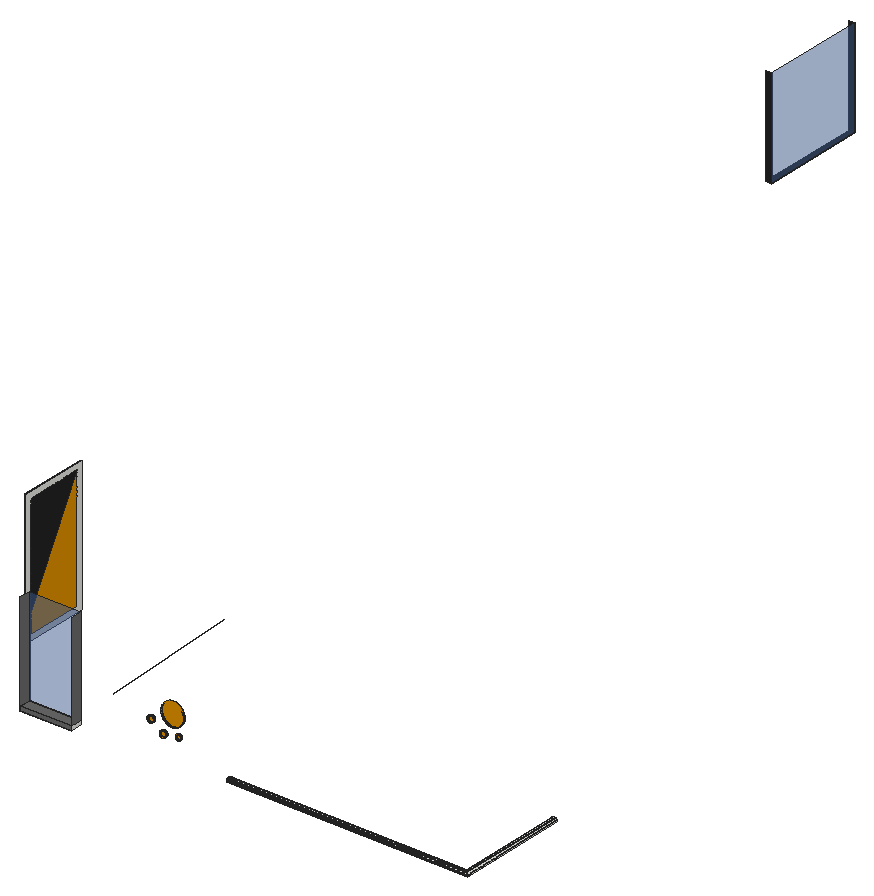
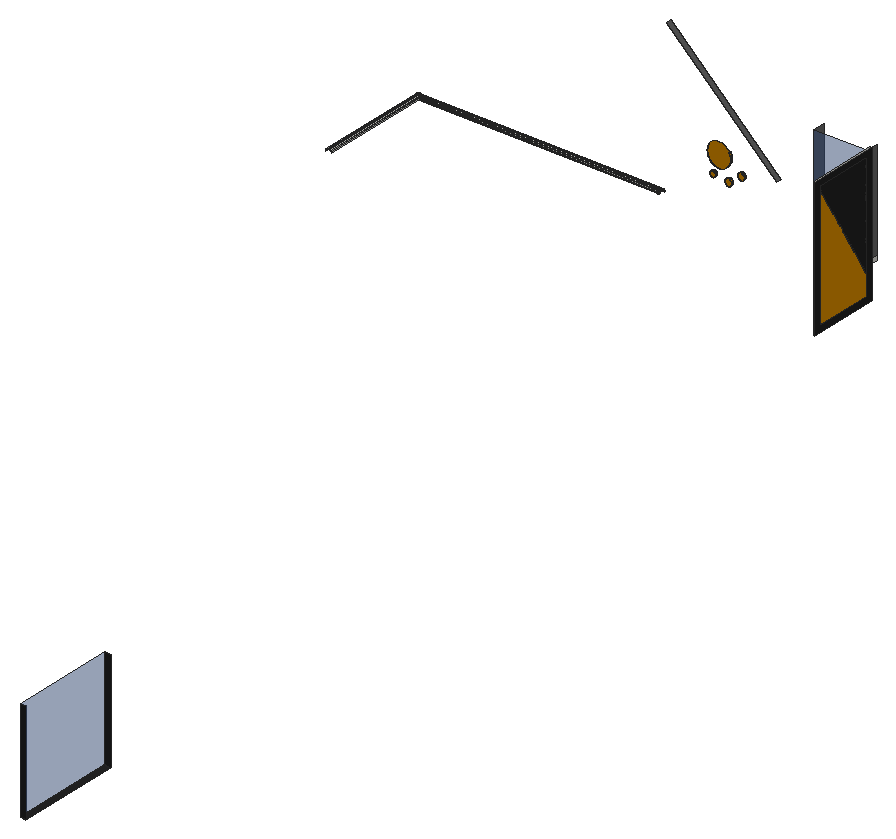
# SketchUp Ruby script. Lengths in inches.
U = 1.inch
M = Sketchup.active_model
def pt(a) = Geom::Point3d.new(a.map { |v| v * U })
def face(e, loops, mat)
  f = e.add_face(loops[0].map { |a| pt(a) })
  loops[1..].each { |l| e.add_face(l.map { |a| pt(a) }).erase! }
  f.material = f.back_material = mat if mat
  f
end
# faces: each face lists its corners as indices into pts; further lists are holes
def faces(e, pts, list, mat = nil) = list.each { |f| face(e, (f[0].is_a?(Array) ? f : [f]).map { |l| l.map { |i| pts[i] } }, mat) }
# xy, xz, yz: faces in a plane at the given z, y or x. An outline is a flat list of corners, or four numbers for a rectangle; further outlines are holes
def ring(l) = l.size == 4 ? [[l[0], l[1]], [l[2], l[1]], [l[2], l[3]], [l[0], l[3]]] : l.each_slice(2).to_a
def flat(e, list, mat, &to3) = list.each { |f| face(e, (f[0].is_a?(Array) ? f : [f]).map { |l| ring(l).map { |u, v| to3.(u, v) } }, mat) }
def xy(e, z, list, mat = nil) = flat(e, list, mat) { |x, y| [x, y, z] }
def xz(e, y, list, mat = nil) = flat(e, list, mat) { |x, z| [x, y, z] }
def yz(e, x, list, mat = nil) = flat(e, list, mat) { |y, z| [x, y, z] }
def lines(e, pts, list) = list.each { |a, b| e.add_line(pt(pts[a]), pt(pts[b])) }
# prism: a flat outline (further loops are holes) pulled along v
def prism(e, loops, v, mat = nil)
  f = face(e, loops, mat); d = Geom::Vector3d.new(v.map { |x| x * U })
  f.pushpull(f.normal.samedirection?(d) ? d.length : -d.length)
end
def box(e, o, s, mat = nil) = prism(e, [[o, [o[0] + s[0], o[1], o[2]], [o[0] + s[0], o[1] + s[1], o[2]], [o[0], o[1] + s[1], o[2]]]], [0, 0, s[2]], mat)
def at(x, y, z, deg = 0) = Geom::Transformation.translation(pt([x, y, z])) * Geom::Transformation.rotation(ORIGIN, Z_AXIS, deg.degrees)
def axes(o, x, y, z) = Geom::Transformation.new([*x, 0, *y, 0, *z, 0, *pt(o).to_a, 1])
def part(name) = M.definitions.add(name)
# library, detail: a bought-in or finely detailed component or shape, given as its bounding box
def library(name, o, s) = part(name).tap { |d| box(d.entities, o, s) }
def detail(e, o, s) = box(e.add_group.entities, o, s)
def put(e, d, t, mat = nil) = e.add_instance(d, t).tap { |i| i.material = mat if mat }
def group(e, t, mat = nil) = e.add_group.tap { |g| g.transformation = t; g.material = mat if mat }.entities
root = M.entities
M.materials.add("[0038_Orange]").color = [221, 143, 0]
M.materials.add("[0134_DimGray]").color = [105, 105, 105]
M.materials.add("[0135_DarkGray]").color = [35, 35, 35]
M.materials.add("[0136_Charcoal]").color = [35, 35, 35]
M.materials.add("[Translucent Glass Blue]").color = [73, 109, 173]
M.materials["[Translucent Glass Blue]"].alpha = 0.5
xy(root,610,[[174,12,282,36]],"[0134_DimGray]")
xy(root,618,[[174,12,282,36]],"[0134_DimGray]")
xy(root,635.9,[[69,155.11,72,299.92]],"[0135_DarkGray]")
xy(root,642.81,[[60,2106,72,2322]],"[0136_Charcoal]")
xy(root,647.9,[[69,167.11,72,287.92]],"[0135_DarkGray]")
xy(root,652.35,[[460.54,27,461.42,30]],"[0038_Orange]")
xy(root,666.32,[[460.54,27,461.42,30]],"[0038_Orange]")
xy(root,671.83,[[434.44,27,435.32,30]],"[0038_Orange]")
xy(root,685.81,[[434.44,27,435.32,30]],"[0038_Orange]")
xz(root,12,[[174,610,282,618]],"[0134_DimGray]")
xz(root,30,[[460.54,652.35,461.42,652.35,462.29,652.46,463.14,652.68,463.96,653,464.73,653.43,465.4375,653.95,466.08,654.55,466.64,655.22,467.11,655.97,467.48,656.76,467.76,657.6,467.92,658.46,467.98,659.34,467.92,660.22,467.76,661.08,467.48,661.92,467.11,662.71,466.64,663.45,466.08,664.13,465.4375,664.73,464.73,665.25,463.96,665.67,463.14,666,462.29,666.21,461.42,666.32,460.54,666.32,459.66,666.21,458.8125,666,458,665.67,457.22,665.25,456.51,664.73,455.875,664.13,455.3125,663.45,454.84,662.71,454.47,661.92,454.2,661.08,454.03,660.22,453.98,659.34,454.03,658.46,454.2,657.6,454.47,656.76,454.84,655.97,455.3125,655.22,455.875,654.55,456.51,653.95,457.22,653.43,458,653,458.8125,652.68,459.66,652.46],[492.87,657.98,493.49,658.01,494.11,658.11,494.72,658.27,495.31,658.5,495.87,658.78,496.39,659.12,496.88,659.52,497.33,659.96,497.72,660.45,498.07,660.97,498.35,661.53,498.58,662.12,498.74,662.72,498.84,663.35,498.87,663.97,498.84,664.6,498.74,665.22,498.58,665.83,498.36,666.41,498.07,666.97,497.73,667.5,497.34,667.99,496.89,668.43,496.41,668.83,495.88,669.17,495.32,669.46,494.73,669.68,494.13,669.85,493.51,669.95,492.88,669.98,492.25,669.95,491.63,669.85,491.03,669.6875,490.44,669.46,489.88,669.18,489.35,668.84,488.86,668.44,488.42,668,488.02,667.51,487.68,666.99,487.39,666.43,487.17,665.84,487.01,665.24,486.91,664.61,486.87,663.99,486.9,663.36,487,662.74,487.16,662.13,487.39,661.55,487.67,660.99,488.01,660.46,488.41,659.97,488.85,659.53,489.34,659.13,489.87,658.79,490.43,658.5,491.01,658.28,491.62,658.11,492.24,658.01],[434.44,671.83,435.32,671.83,436.19,671.94,437.05,672.16,437.86,672.49,438.63,672.91,439.35,673.43,439.99,674.03,440.55,674.7,441.02,675.45,441.39,676.24,441.66,677.08,441.83,677.94,441.88,678.82,441.83,679.7,441.66,680.56,441.39,681.4,441.02,682.19,440.55,682.93,439.99,683.61,439.35,684.21,438.63,684.73,437.86,685.15,437.05,685.48,436.19,685.7,435.32,685.81,434.44,685.81,433.57,685.7,432.72,685.48,431.9,685.15,431.13,684.73,430.42,684.21,429.78,683.61,429.22,682.93,428.75,682.19,428.375,681.4,428.1,680.56,427.9375,679.7,427.88,678.82,427.9375,677.94,428.1,677.08,428.375,676.24,428.75,675.45,429.22,674.7,429.78,674.03,430.42,673.43,431.13,672.91,431.9,672.49,432.72,672.16,433.57,671.94],[480.75,679.13,483.26,679.3,485.73,679.73,488.15,680.41,490.48,681.35,492.71,682.52,494.79,683.92,496.72,685.53,498.47,687.33,500.02,689.31,501.36,691.43,502.47,693.6875,503.34,696.04,503.95,698.48,504.31,700.97,504.4,703.48,504.24,705.98,503.81,708.46,503.12,710.875,502.1875,713.21,501.02,715.43,499.62,717.52,498.01,719.45,496.21,721.2,494.23,722.75,492.11,724.09,489.85,725.19,487.49,726.0625,485.06,726.68,482.57,727.03,480.06,727.13,477.55,726.96,475.08,726.53,472.66,725.85,470.33,724.91,468.11,723.74,466.02,722.34,464.09,720.73,462.34,718.93,460.79,716.96,459.45,714.83,458.34,712.57,457.48,710.22,456.86,707.78,456.5,705.29,456.41,702.78,456.58,700.28,457.01,697.8,457.69,695.39,458.625,693.05,459.8,690.83,461.2,688.75,462.8,686.82,464.61,685.07,466.58,683.51,468.71,682.18,470.96,681.07,473.32,680.2,475.76,679.59,478.24,679.23]],"[0038_Orange]")
xz(root,36,[[174,610,282,618]])
xz(root,36,[[174,618,282,822]],"[Translucent Glass Blue]")
xz(root,155.11,[[69,635.9,72,915.4]],"[0135_DarkGray]")
xz(root,167.11,[[69,647.9,72,903.4]],"[0135_DarkGray]")
xz(root,287.92,[[69,647.9,72,903.4]],"[0135_DarkGray]")
xz(root,299.92,[[69,635.9,72,915.4]],"[0135_DarkGray]")
xz(root,2106,[[60,642.81,72,849.4]],"[0135_DarkGray]")
xz(root,2322,[[60,642.81,72,849.4]],"[0135_DarkGray]")
yz(root,69,[[[155.11,635.9,299.92,915.4],[167.11,647.9,287.92,903.4]]],"[0135_DarkGray]")
yz(root,72,[[[155.11,635.9,299.92,915.4],[167.11,647.9,287.92,903.4]]])
yz(root,72,[[167.11,647.9,167.11,690.375,287.92,903.4,287.92,647.9]],"[0038_Orange]")
yz(root,72,[[167.11,690.375,167.11,903.4,287.92,903.4]],"[0135_DarkGray]")
yz(root,72,[[2106,642.81,2322,849.4]],"[Translucent Glass Blue]")
yz(root,174,[[12,610,36,618]])
yz(root,174,[[12,618,36,822]],"[0134_DimGray]")
yz(root,282,[[12,610,36,618]])
yz(root,282,[[12,618,36,822]],"[0134_DimGray]")
p = [[1086,42,606],[1085.8,42.2,607.55],[582,42.2,607.55],[582,42,606],[1086,276,606],[1085.8,276,607.55],
  [1074.2,53.8,607.55],[1074,54,606],[582,54,606],[582,53.8,607.55],[1074.2,276,607.55],[1074,276,606],
  [1085.2,42.8,609],[582,42.8,609],[1085.2,276,609],[1074.8,53.2,609],[582,53.2,609],[1074.8,276,609],
  [1084.24,43.76,610.24],[582,43.76,610.24],[1084.24,276,610.24],[1075.76,52.24,610.24],[582,52.24,610.24],[1075.76,276,610.24],
  [1083,45,611.2],[582,45,611.2],[1083,276,611.2],[1077,51,611.2],[582,51,611.2],[1077,276,611.2],
  [1081.55,46.45,611.8],[582,46.45,611.8],[1081.55,276,611.8],[1078.45,49.55,611.8],[582,49.55,611.8],[1078.45,276,611.8],
  [1080,48,612],[582,48,612],[1080,276,612],[459.66,27,652.46],[460.54,27,652.35],[460.54,30,652.35],
  [459.66,30,652.46],[461.42,27,652.35],[462.29,27,652.46],[462.29,30,652.46],[461.42,30,652.35],[458.8125,27,652.68],
  [458.8125,30,652.68],[463.14,27,652.68],[463.14,30,652.68],[458,27,653],[458,30,653],[463.96,27,653],
  [463.96,30,653],[457.22,27,653.43],[457.22,30,653.43],[464.73,27,653.43],[464.73,30,653.43],[456.51,27,653.95],
  [456.51,30,653.95],[465.4375,27,653.95],[465.4375,30,653.95],[455.875,27,654.55],[455.875,30,654.55],[466.08,27,654.55],
  [466.08,30,654.55],[455.3125,27,655.22],[455.3125,30,655.22],[466.64,27,655.22],[466.64,30,655.22],[454.84,27,655.97],
  [454.84,30,655.97],[467.11,27,655.97],[467.11,30,655.97],[454.47,27,656.76],[454.47,30,656.76],[467.48,27,656.76],
  [467.48,30,656.76],[454.2,27,657.6],[454.2,30,657.6],[467.76,27,657.6],[467.76,30,657.6],[454.03,27,658.46],
  [454.03,30,658.46],[467.92,27,658.46],[467.92,30,658.46],[491.62,27,658.11],[492.24,27,658.01],[492.24,30,658.01],
  [491.62,30,658.11],[492.87,27,657.98],[492.87,30,657.98],[493.49,27,658.01],[493.49,30,658.01],[494.11,27,658.11],
  [494.11,30,658.11],[491.01,27,658.28],[491.01,30,658.28],[494.72,27,658.27],[494.72,30,658.27],[490.43,27,658.5],
  [490.43,30,658.5],[495.31,27,658.5],[495.31,30,658.5],[453.98,27,659.34],[453.98,30,659.34],[467.98,27,659.34],
  [467.98,30,659.34],[489.87,27,658.79],[489.87,30,658.79],[495.87,27,658.78],[495.87,30,658.78],[489.34,27,659.13],
  [489.34,30,659.13],[496.39,27,659.12],[496.39,30,659.12],[488.85,27,659.53],[488.85,30,659.53],[496.88,27,659.52],
  [496.88,30,659.52],[454.03,27,660.22],[454.03,30,660.22],[467.92,27,660.22],[467.92,30,660.22],[488.41,27,659.97],
  [488.41,30,659.97],[497.33,27,659.96],[497.33,30,659.96],[488.01,27,660.46],[488.01,30,660.46],[497.72,27,660.45],
  [497.72,30,660.45],[454.2,27,661.08],[454.2,30,661.08],[467.76,27,661.08],[467.76,30,661.08],[498.07,27,660.97],
  [498.07,30,660.97],[487.67,27,660.99],[487.67,30,660.99],[487.39,27,661.55],[487.39,30,661.55],[498.35,27,661.53],
  [498.35,30,661.53],[454.47,27,661.92],[454.47,30,661.92],[467.48,27,661.92],[467.48,30,661.92],[487.16,27,662.13],
  [487.16,30,662.13],[498.58,27,662.12],[498.58,30,662.12],[454.84,27,662.71],[454.84,30,662.71],[467.11,27,662.71],
  [467.11,30,662.71],[487,27,662.74],[487,30,662.74],[498.74,27,662.72],[498.74,30,662.72],[455.3125,27,663.45],
  [455.3125,30,663.45],[466.64,27,663.45],[466.64,30,663.45],[486.9,27,663.36],[486.9,30,663.36],[498.84,27,663.35],
  [498.84,30,663.35],[498.87,27,663.97],[498.87,30,663.97],[486.87,27,663.99],[486.87,30,663.99],[455.875,27,664.13],
  [455.875,30,664.13],[466.08,27,664.13],[466.08,30,664.13],[486.91,27,664.61],[486.91,30,664.61],[498.84,27,664.6],
  [498.84,30,664.6],[456.51,27,664.73],[456.51,30,664.73],[465.4375,27,664.73],[465.4375,30,664.73],[487.01,27,665.24],
  [487.01,30,665.24],[498.74,27,665.22],[498.74,30,665.22],[457.22,27,665.25],[457.22,30,665.25],[464.73,27,665.25],
  [464.73,30,665.25],[458,27,665.67],[458,30,665.67],[463.96,27,665.67],[463.96,30,665.67],[487.17,27,665.84],
  [487.17,30,665.84],[498.58,27,665.83],[498.58,30,665.83],[458.8125,27,666],[458.8125,30,666],[463.14,27,666],
  [463.14,30,666],[487.39,27,666.43],[487.39,30,666.43],[498.36,27,666.41],[498.36,30,666.41],[459.66,27,666.21],
  [459.66,30,666.21],[462.29,27,666.21],[462.29,30,666.21],[460.54,27,666.32],[460.54,30,666.32],[461.42,27,666.32],
  [461.42,30,666.32],[487.68,27,666.99],[487.68,30,666.99],[498.07,27,666.97],[498.07,30,666.97],[488.02,27,667.51],
  [488.02,30,667.51],[497.73,27,667.5],[497.73,30,667.5],[488.42,27,668],[488.42,30,668],[497.34,27,667.99],
  [497.34,30,667.99],[488.86,27,668.44],[488.86,30,668.44],[496.89,27,668.43],[496.89,30,668.43],[489.35,27,668.84],
  [489.35,30,668.84],[496.41,27,668.83],[496.41,30,668.83],[489.88,27,669.18],[489.88,30,669.18],[495.88,27,669.17],
  [495.88,30,669.17],[490.44,27,669.46],[490.44,30,669.46],[495.32,27,669.46],[495.32,30,669.46],[491.03,27,669.6875],
  [491.03,30,669.6875],[494.73,27,669.68],[494.73,30,669.68],[491.63,27,669.85],[491.63,30,669.85],[494.13,27,669.85],
  [494.13,30,669.85],[493.51,27,669.95],[493.51,30,669.95],[492.25,27,669.95],[492.25,30,669.95],[492.88,27,669.98],
  [492.88,30,669.98],[433.57,27,671.94],[434.44,27,671.83],[434.44,30,671.83],[433.57,30,671.94],[435.32,27,671.83],
  [436.19,27,671.94],[436.19,30,671.94],[435.32,30,671.83],[432.72,27,672.16],[432.72,30,672.16],[437.05,27,672.16],
  [437.05,30,672.16],[431.9,27,672.49],[431.9,30,672.49],[437.86,27,672.49],[437.86,30,672.49],[431.13,27,672.91],
  [431.13,30,672.91],[438.63,27,672.91],[438.63,30,672.91],[430.42,27,673.43],[430.42,30,673.43],[439.35,27,673.43],
  [439.35,30,673.43],[429.78,27,674.03],[429.78,30,674.03],[439.99,27,674.03],[439.99,30,674.03],[429.22,27,674.7],
  [429.22,30,674.7],[440.55,27,674.7],[440.55,30,674.7],[428.75,27,675.45],[428.75,30,675.45],[441.02,27,675.45],
  [441.02,30,675.45],[428.375,27,676.24],[428.375,30,676.24],[441.39,27,676.24],[441.39,30,676.24],[428.1,27,677.08],
  [428.1,30,677.08],[441.66,27,677.08],[441.66,30,677.08],[427.9375,27,677.94],[427.9375,30,677.94],[441.83,27,677.94],
  [441.83,30,677.94],[427.88,27,678.82],[427.88,30,678.82],[441.88,27,678.82],[441.88,30,678.82],[427.9375,27,679.7],
  [427.9375,30,679.7],[441.83,27,679.7],[441.83,30,679.7],[478.24,27,679.23],[480.75,27,679.13],[480.75,30,679.13],
  [478.24,30,679.23],[483.26,27,679.3],[483.26,30,679.3],[475.76,27,679.59],[475.76,30,679.59],[485.73,27,679.73],
  [485.73,30,679.73],[473.32,27,680.2],[473.32,30,680.2],[428.1,27,680.56],[428.1,30,680.56],[441.66,27,680.56],
  [441.66,30,680.56],[488.15,27,680.41],[488.15,30,680.41],[470.96,27,681.07],[470.96,30,681.07],[490.48,27,681.35],
  [490.48,30,681.35],[428.375,27,681.4],[428.375,30,681.4],[441.39,27,681.4],[441.39,30,681.4],[468.71,27,682.18],
  [468.71,30,682.18],[492.71,27,682.52],[492.71,30,682.52],[428.75,27,682.19],[428.75,30,682.19],[441.02,27,682.19],
  [441.02,30,682.19],[429.22,27,682.93],[429.22,30,682.93],[440.55,27,682.93],[440.55,30,682.93],[466.58,27,683.51],
  [466.58,30,683.51],[494.79,27,683.92],[494.79,30,683.92],[429.78,27,683.61],[429.78,30,683.61],[439.99,27,683.61],
  [439.99,30,683.61],[464.61,27,685.07],[464.61,30,685.07],[430.42,27,684.21],[430.42,30,684.21],[439.35,27,684.21],
  [439.35,30,684.21],[496.72,27,685.53],[496.72,30,685.53],[431.13,27,684.73],[431.13,30,684.73],[438.63,27,684.73],
  [438.63,30,684.73],[431.9,27,685.15],[431.9,30,685.15],[437.86,27,685.15],[437.86,30,685.15],[462.8,27,686.82],
  [462.8,30,686.82],[432.72,27,685.48],[432.72,30,685.48],[437.05,27,685.48],[437.05,30,685.48],[433.57,27,685.7],
  [433.57,30,685.7],[436.19,27,685.7],[436.19,30,685.7],[498.47,27,687.33],[498.47,30,687.33],[434.44,27,685.81],
  [434.44,30,685.81],[435.32,27,685.81],[435.32,30,685.81],[461.2,27,688.75],[461.2,30,688.75],[500.02,27,689.31],
  [500.02,30,689.31],[459.8,27,690.83],[459.8,30,690.83],[501.36,27,691.43],[501.36,30,691.43],[458.625,27,693.05],
  [458.625,30,693.05],[502.47,27,693.6875],[502.47,30,693.6875],[457.69,27,695.39],[457.69,30,695.39],[503.34,27,696.04],
  [503.34,30,696.04],[457.01,27,697.8],[457.01,30,697.8],[503.95,27,698.48],[503.95,30,698.48],[456.58,27,700.28],
  [456.58,30,700.28],[504.31,27,700.97],[504.31,30,700.97],[582,36,912],[357.71,36,698.8],[357.71,27,698.8],
  [582,27,912],[456.41,27,702.78],[456.41,30,702.78],[504.4,27,703.48],[504.4,30,703.48],[456.5,27,705.29],
  [456.5,30,705.29],[504.24,27,705.98],[504.24,30,705.98],[456.86,27,707.78],[456.86,30,707.78],[503.81,27,708.46],
  [503.81,30,708.46],[457.48,27,710.22],[457.48,30,710.22],[503.12,27,710.875],[503.12,30,710.875],[458.34,27,712.57],
  [458.34,30,712.57],[502.1875,27,713.21],[502.1875,30,713.21],[459.45,27,714.83],[459.45,30,714.83],[501.02,27,715.43],
  [501.02,30,715.43]]
faces(root,p,[[0,1,2,3],[4,5,1,0],[6,7,8,9],[10,11,7,6],[1,12,13,2],[5,14,12,1],[15,6,9,16],[17,10,6,15],
  [12,18,19,13],[14,20,18,12],[21,15,16,22],[23,17,15,21],[18,24,25,19],[20,26,24,18],[27,21,22,28],[29,23,21,27],
  [24,30,31,25],[26,32,30,24],[33,27,28,34],[35,29,27,33],[30,36,37,31],[32,38,36,30],[36,33,34,37],[38,35,33,36]])
faces(root,p,[[39,40,41,42],[43,44,45,46],[47,39,42,48],[44,49,50,45],[51,47,48,52],[49,53,54,50],[55,51,52,56],[53,57,58,54],
  [59,55,56,60],[57,61,62,58],[63,59,60,64],[61,65,66,62],[67,63,64,68],[65,69,70,66],[71,67,68,72],[69,73,74,70],
  [75,71,72,76],[73,77,78,74],[79,75,76,80],[77,81,82,78],[83,79,80,84],[81,85,86,82],[87,88,89,90],[88,91,92,89],
  [91,93,94,92],[93,95,96,94],[97,87,90,98],[95,99,100,96],[101,97,98,102],[99,103,104,100],[105,83,84,106],[85,107,108,86],
  [109,101,102,110],[103,111,112,104],[113,109,110,114],[111,115,116,112],[117,113,114,118],[115,119,120,116],[121,105,106,122],[107,123,124,108],
  [125,117,118,126],[119,127,128,120],[129,125,126,130],[127,131,132,128],[133,121,122,134],[123,135,136,124],[131,137,138,132],[139,129,130,140],
  [141,139,140,142],[137,143,144,138],[145,133,134,146],[135,147,148,136],[149,141,142,150],[143,151,152,144],[153,145,146,154],[147,155,156,148],
  [157,149,150,158],[151,159,160,152],[161,153,154,162],[155,163,164,156],[165,157,158,166],[159,167,168,160],[167,169,170,168],[171,165,166,172],
  [173,161,162,174],[163,175,176,164],[177,171,172,178],[169,179,180,170],[181,173,174,182],[175,183,184,176],[185,177,178,186],[179,187,188,180],
  [189,181,182,190],[183,191,192,184],[193,189,190,194],[191,195,196,192],[197,185,186,198],[187,199,200,188],[201,193,194,202],[195,203,204,196],
  [205,197,198,206],[199,207,208,200],[209,201,202,210],[203,211,212,204],[213,209,210,214],[211,215,216,212],[217,205,206,218],[207,219,220,208],
  [221,217,218,222],[219,223,224,220],[225,221,222,226],[223,227,228,224],[229,225,226,230],[227,231,232,228],[233,229,230,234],[231,235,236,232],
  [237,233,234,238],[235,239,240,236],[241,237,238,242],[239,243,244,240],[245,241,242,246],[243,247,248,244],[249,245,246,250],[247,251,252,248],
  [251,253,254,252],[255,249,250,256],[257,255,256,258],[253,257,258,254],[259,260,261,262],[263,264,265,266],[267,259,262,268],[264,269,270,265],
  [271,267,268,272],[269,273,274,270],[275,271,272,276],[273,277,278,274],[279,275,276,280],[277,281,282,278],[283,279,280,284],[281,285,286,282],
  [287,283,284,288],[285,289,290,286],[291,287,288,292],[289,293,294,290],[295,291,292,296],[293,297,298,294],[299,295,296,300],[297,301,302,298],
  [303,299,300,304],[301,305,306,302],[307,303,304,308],[305,309,310,306],[311,307,308,312],[309,313,314,310],[315,316,317,318],[316,319,320,317],
  [321,315,318,322],[319,323,324,320],[325,321,322,326],[327,311,312,328],[313,329,330,314],[323,331,332,324],[333,325,326,334],[331,335,336,332],
  [337,327,328,338],[329,339,340,330],[341,333,334,342],[335,343,344,336],[345,337,338,346],[339,347,348,340],[349,345,346,350],[347,351,352,348],
  [353,341,342,354],[343,355,356,344],[357,349,350,358],[351,359,360,352],[361,353,354,362],[363,357,358,364],[359,365,366,360],[355,367,368,356],
  [369,363,364,370],[365,371,372,366],[373,369,370,374],[371,375,376,372],[377,361,362,378],[379,373,374,380],[375,381,382,376],[383,379,380,384],
  [381,385,386,382],[367,387,388,368],[389,383,384,390],[385,391,392,386],[393,377,378,394],[387,395,396,388],[397,393,394,398],[395,399,400,396],
  [401,397,398,402],[399,403,404,400],[405,401,402,406],[403,407,408,404],[409,405,406,410],[407,411,412,408],[413,409,410,414],[411,415,416,412],
  [421,413,414,422],[415,423,424,416],[425,421,422,426],[423,427,428,424],[429,425,426,430],[427,431,432,428],[433,429,430,434],[431,435,436,432],
  [437,433,434,438],[435,439,440,436],[441,437,438,442],[439,443,444,440]],"[0038_Orange]")
faces(root,p,[[417,418,419,420]],"[0134_DimGray]")
